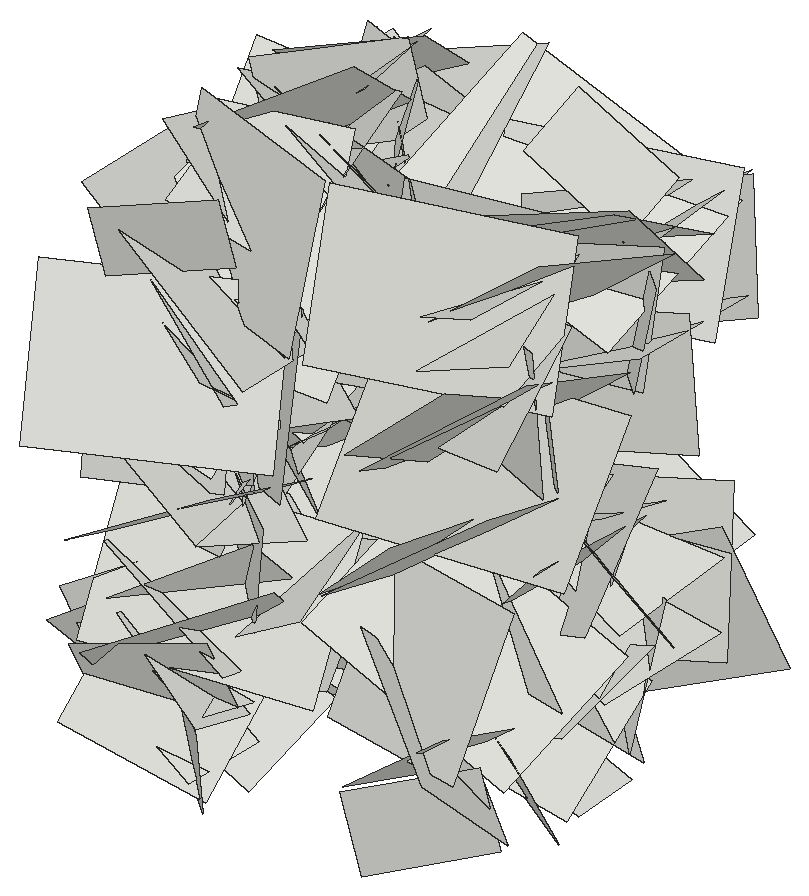
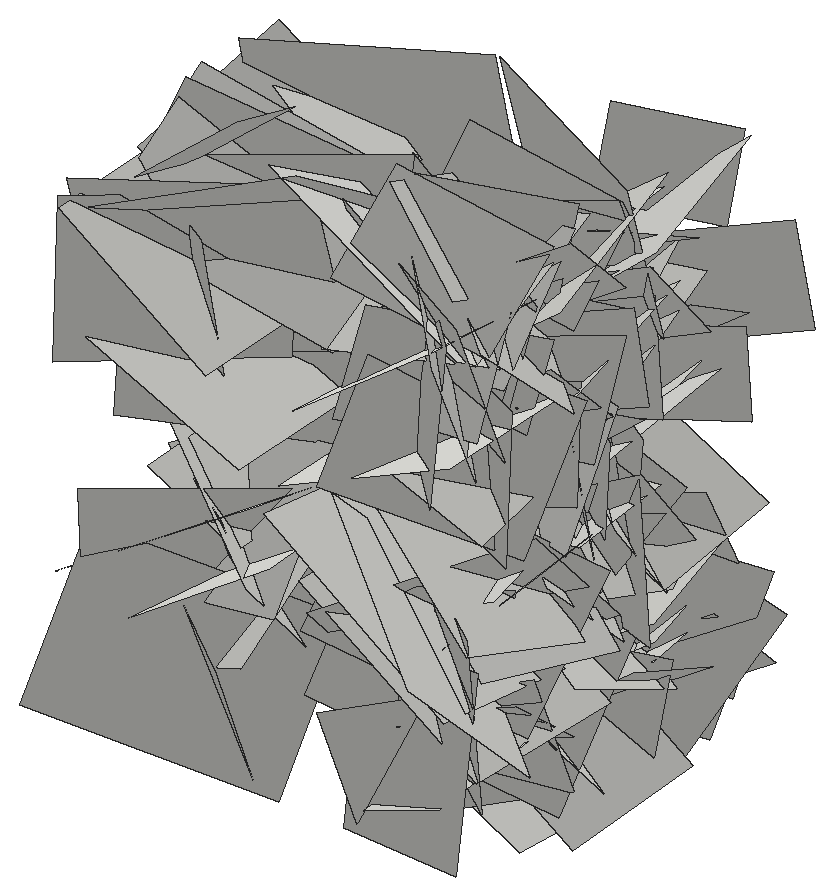
# SketchUp Ruby script. Lengths in inches.
U = 1.inch
M = Sketchup.active_model
def pt(a) = Geom::Point3d.new(a.map { |v| v * U })
def face(e, loops, mat)
  f = e.add_face(loops[0].map { |a| pt(a) })
  loops[1..].each { |l| e.add_face(l.map { |a| pt(a) }).erase! }
  f.material = f.back_material = mat if mat
  f
end
# faces: each face lists its corners as indices into pts; further lists are holes
def faces(e, pts, list, mat = nil) = list.each { |f| face(e, (f[0].is_a?(Array) ? f : [f]).map { |l| l.map { |i| pts[i] } }, mat) }
# xy, xz, yz: faces in a plane at the given z, y or x. An outline is a flat list of corners, or four numbers for a rectangle; further outlines are holes
def ring(l) = l.size == 4 ? [[l[0], l[1]], [l[2], l[1]], [l[2], l[3]], [l[0], l[3]]] : l.each_slice(2).to_a
def flat(e, list, mat, &to3) = list.each { |f| face(e, (f[0].is_a?(Array) ? f : [f]).map { |l| ring(l).map { |u, v| to3.(u, v) } }, mat) }
def xy(e, z, list, mat = nil) = flat(e, list, mat) { |x, y| [x, y, z] }
def xz(e, y, list, mat = nil) = flat(e, list, mat) { |x, z| [x, y, z] }
def yz(e, x, list, mat = nil) = flat(e, list, mat) { |y, z| [x, y, z] }
def lines(e, pts, list) = list.each { |a, b| e.add_line(pt(pts[a]), pt(pts[b])) }
# prism: a flat outline (further loops are holes) pulled along v
def prism(e, loops, v, mat = nil)
  f = face(e, loops, mat); d = Geom::Vector3d.new(v.map { |x| x * U })
  f.pushpull(f.normal.samedirection?(d) ? d.length : -d.length)
end
def box(e, o, s, mat = nil) = prism(e, [[o, [o[0] + s[0], o[1], o[2]], [o[0] + s[0], o[1] + s[1], o[2]], [o[0], o[1] + s[1], o[2]]]], [0, 0, s[2]], mat)
def at(x, y, z, deg = 0) = Geom::Transformation.translation(pt([x, y, z])) * Geom::Transformation.rotation(ORIGIN, Z_AXIS, deg.degrees)
def axes(o, x, y, z) = Geom::Transformation.new([*x, 0, *y, 0, *z, 0, *pt(o).to_a, 1])
def part(name) = M.definitions.add(name)
# library, detail: a bought-in or finely detailed component or shape, given as its bounding box
def library(name, o, s) = part(name).tap { |d| box(d.entities, o, s) }
def detail(e, o, s) = box(e.add_group.entities, o, s)
def put(e, d, t, mat = nil) = e.add_instance(d, t).tap { |i| i.material = mat if mat }
def group(e, t, mat = nil) = e.add_group.tap { |g| g.transformation = t; g.material = mat if mat }.entities
root = M.entities
c1 = part("Component\#6")
p = [[0.01,0,0],[0,3.24,4.54],[4.32,3.24,4.54],[4.33,0,0]]
faces(c1.entities,p,[[0,1,2,3]])
put(root,c1,axes([24.34,175.72,36.8],[-0.15665,0.75943,0.7145],[-0.11122,0.70715,-0.77331],[1.09966,0.17971,0.02357]))
put(root,c1,axes([28.31,175.72,36.8],[0.15665,0.75943,0.7145],[0.11122,0.70715,-0.77331],[-1.09966,0.17971,0.02357]))
put(root,c1,axes([24.34,182.09,31.375],[0.0562,-0.72005,0.10613],[0.07977,0.11126,0.71729],[0.76737,0.04117,-0.08234]))
put(root,c1,axes([28.31,170.91,25.11],[-0.00896,0.33986,-0.6335],[-0.15678,-0.62081,-0.33108],[-0.74574,0.12644,0.07722]))
put(root,c1,axes([28.31,181.67,36.78],[0.05967,0.56874,-0.94691],[0.29528,-0.9248,-0.5389],[-1.13301,-0.21107,-0.19031]))
put(root,c1,axes([28.31,180.66,33.34],[0.08177,-0.45253,0.73357],[-0.03972,0.73405,0.45677],[-0.91278,-0.07248,0.04584]))
put(root,c1,axes([24.34,176.52,27.27],[0.06139,-0.83333,-0.30669],[-0.14477,-0.31205,0.82208],[0.93005,0.00643,0.1482]))
put(root,c1,axes([24.34,174.67,32.54],[-0.17055,0.3665,0.95024],[-0.03456,0.95968,-0.37566],[1.07902,0.08867,0.13816]))
put(root,c1,axes([24.34,177.99,23.55],[0.04107,0.5427,0.4395],[0.20397,0.41484,-0.52921],[0.71159,-0.15024,0.12632]))
put(root,c1,axes([24.34,177.89,30.77],[0.05678,-0.11721,0.8526],[-0.09083,0.84928,0.12214],[0.90772,0.09231,-0.04111]))
put(root,c1,axes([24.34,174.875,32.24],[0.12053,0.70886,0.38052],[-0.08644,0.39248,-0.70676],[0.84842,-0.06072,-0.12606]))
put(root,c1,axes([24.34,176.26,32.94],[0.03084,0.60524,0.59943],[-0.03406,0.60013,-0.60439],[0.90231,0.00196,-0.0433]))
put(root,c1,axes([24.34,169.05,21.98],[0.04882,0.58162,0.59704],[-0.02934,0.59868,-0.58109],[0.88303,-0.01226,-0.05232]))
put(root,c1,axes([24.34,171.18,26.98],[-0.09963,0.88743,-0.23237],[0.05305,-0.22828,-0.89204],[0.97094,0.10354,0.02489]))
put(root,c1,axes([24.34,174.16,29.86],[0.19319,0.59277,-0.26834],[0.07097,-0.29428,-0.60458],[0.68606,-0.13648,0.1381]))
put(root,c1,axes([28.31,171.52,27.71],[0.03995,0.48298,0.66079],[0.01207,0.66111,-0.48387],[-0.8675,0.03144,0.0237]))
put(root,c1,axes([24.34,174.95,31.63],[0.12097,-0.07785,-0.70642],[0.09105,-0.70871,0.09198],[0.74781,0.09888,0.10307]))
put(root,c1,axes([24.34,178.01,36.42],[0.04909,-0.68925,0.58112],[-0.09024,0.57594,0.68989],[0.95135,0.0902,0.03545]))
put(root,c1,axes([24.34,172,20.82],[-0.19013,-0.4174,1.11707],[-0.18593,1.12659,0.39279],[1.25031,0.10406,0.22828]))
put(root,c1,axes([28.31,172.01,32.68],[-0.01531,-0.04852,-0.71126],[-0.05574,-0.70939,0.04946],[-0.75363,0.05345,0.01079]))
put(root,c1,axes([24.34,184.3,37.98],[-0.01849,-0.42221,-1.00939],[-0.24573,-0.98518,0.41609],[1.13346,-0.22047,0.07374]))
put(root,c1,axes([24.34,175.14,30.45],[-0.22771,0.17317,-1.07869],[0.0194,-1.09862,-0.18001],[1.15789,0.05246,-0.20912]))
put(root,c1,axes([28.31,173.36,27.66],[0.12062,0.63946,0.63128],[0.06443,0.62939,-0.6485],[-0.9503,0.12384,0.03616]))
put(root,c1,axes([28.31,173.29,20.87],[-0.09428,-0.62013,-0.08152],[-0.03551,-0.0775,0.6261],[-0.66205,0.09247,-0.02197]))
put(root,c1,axes([24.34,180.04,24.28],[0.15161,0.71603,-0.23582],[0.04269,-0.24694,-0.72538],[0.79796,-0.12284,0.08362]))
put(root,c1,axes([24.34,178.05,19.9375],[-0.14578,-1.0409,0.22357],[-0.02192,0.228,1.04879],[1.1283,-0.13006,0.04926]))
put(root,c1,axes([24.34,171.36,22.89],[0.02535,0.88672,0.32576],[-0.06435,0.32663,-0.88464],[0.99927,-0.00146,-0.06523]))
put(root,c1,axes([24.34,176.41,32.2],[0.11408,-0.0942,-0.79779],[0.0272,-0.8041,0.09841],[0.85109,0.03832,0.10379]))
put(root,c1,axes([28.31,177.7,39.03],[0.08239,-0.33737,-0.64844],[-0.10668,-0.65083,0.32654],[-0.76743,0.05425,-0.11501]))
put(root,c1,axes([24.34,181.8125,37.17],[-0.0246,-0.63961,0.56311],[0.17949,0.54862,0.63013],[0.88529,-0.129,-0.11211]))
put(root,c1,axes([24.34,173.5,20.5],[-0.29119,-0.77592,0.90535],[0.00734,0.92801,0.79744],[1.26387,-0.18415,0.20396]))
put(root,c1,axes([24.34,172.625,27.43],[-0.01975,0.58315,0.74345],[0.01761,0.74368,-0.58292],[1.00141,-0.00157,0.02491]))
put(root,c1,axes([24.34,172.13,35.78],[0.07615,0.65901,-0.5201],[0.04859,-0.52431,-0.658],[0.88857,-0.02781,0.08055]))
put(root,c1,axes([24.34,177.13,31.79],[-0.078,-0.30439,1.03044],[-0.07955,1.03178,0.29943],[1.13614,0.05135,0.09171]))
put(root,c1,axes([24.34,182.1,27.04],[-0.18817,-1.1788,-0.21223],[-0.10509,-0.19936,1.19019],[1.26526,-0.19187,0.06729]))
put(root,c1,axes([28.31,180.11,41],[0.0874,0.13713,-0.78202],[0.02965,-0.78624,-0.13492],[-0.84107,-0.01347,-0.08602]))
put(root,c1,axes([28.31,171.42,39.46],[-0.01769,0.21401,-0.61924],[-0.03571,-0.6189,-0.21298],[-0.69357,0.02641,0.02676]))
put(root,c1,axes([28.31,174.375,32.02],[0.18574,0.64681,-0.5499],[0.00393,-0.56207,-0.65994],[-0.8999,0.13105,-0.11638]))
put(root,c1,axes([24.34,167.34,31.77],[-0.2501,0.51374,1.1242],[-0.05799,1.13903,-0.532],[1.3089,0.14863,0.19123]))
put(root,c1,axes([28.31,173.15,22.23],[-0.01199,-0.5915,0.12784],[-0.10227,0.12799,0.58366],[-0.63327,-0.00947,-0.09668]))
put(root,c1,axes([24.34,170.16,39.2],[-0.24703,1.2789,-0.21613],[-0.13589,-0.24123,-1.28918],[1.36812,0.20696,-0.16707]))
put(root,c1,axes([24.34,174.01,26.46],[-0.07872,-0.97306,0.24072],[0.0738,0.23579,0.97461],[1.05998,-0.08868,-0.04998]))
put(root,c1,axes([28.31,173.67,32.24],[0.05341,-0.65994,-0.37026],[0.06447,-0.36634,0.66124],[-0.79951,-0.07362,0.02859]))
put(root,c1,axes([28.31,175.43,34.87],[0.0411,0.62613,0.35799],[0.03637,0.3565,-0.62724],[-0.76365,0.05068,-0.01061]))
put(root,c1,axes([24.34,185.38,28.27],[-0.28552,-0.8956,-0.93898],[-0.07116,-0.9481,0.92355],[1.37362,-0.23528,-0.14733]))
put(root,c1,axes([24.34,182.77,28.15],[-0.11013,-1.0722,-0.31704],[-0.03816,-0.31503,1.07721],[1.18456,-0.10983,0.00522]))
put(root,c1,axes([24.34,176.05,33.17],[0.01986,0.50916,-0.88553],[-0.06176,-0.8837,-0.50934],[1.08099,-0.05984,-0.01283]))
put(root,c1,axes([28.31,182.27,37.76],[0.22679,0.05489,-0.89691],[0.06736,-0.9206,-0.04118],[-0.95012,-0.05216,-0.217]))
put(root,c1,axes([24.34,174.9,23.69],[-0.06803,0.90477,0.33383],[0.16872,0.33992,-0.89067],[1.00823,0.00417,0.17157]))
put(root,c1,axes([28.31,173.11,21.9],[0.05319,-0.68826,0.19248],[0.04456,0.19546,0.68797],[-0.75624,-0.03689,0.05408]))
put(root,c1,axes([28.31,178.15,33.23],[-0.08938,-0.00525,-0.60269],[0.06829,-0.60515,-0.00374],[-0.63521,-0.06432,0.0844]))
put(root,c1,axes([28.31,176.44,21.6],[0.04345,0.60879,-0.00304],[-0.10651,0.00376,-0.60183],[-0.63647,0.04093,0.10051]))
put(root,c1,axes([24.34,183.67,38.38],[0.04708,0.10578,-1.15378],[-0.2342,-1.13267,-0.11235],[1.2056,-0.22416,0.02323]))
put(root,c1,axes([24.34,173.31,35.98],[-0.01252,1.07454,-0.37217],[-0.12805,-0.37127,-1.06811],[1.19858,-0.02844,-0.11799]))
put(root,c1,axes([24.34,174.78,20.26],[0.10048,-0.39109,0.79293],[0.10042,0.79738,0.38196],[0.93179,-0.04376,-0.12667]))
put(root,c1,axes([28.31,180.68,27.18],[0.06604,-0.60003,0.10008],[-0.10227,0.08959,0.59716],[-0.63666,-0.07663,-0.08554]))
put(root,c1,axes([28.31,170.73,19.61],[0.06378,-0.15247,0.68566],[0.07422,0.68605,0.14641],[-0.74085,0.05561,0.0737]))
put(root,c1,axes([24.34,178.01,21.81],[0.00864,0.40014,0.99077],[-0.02339,0.99065,-0.39991],[1.13239,0.01741,-0.01582]))
put(root,c1,axes([28.31,178.13,40.15],[0.04908,0.64392,0.19174],[0.08573,0.18545,-0.64234],[-0.70699,0.06719,-0.06458]))
put(root,c1,axes([24.34,171.95,33.74],[-0.07102,0.70639,0.8167],[0.11892,0.8184,-0.69866],[1.13841,-0.04142,0.12393]))
put(root,c1,axes([28.31,176.07,37.03],[0.15674,-0.62528,-0.09698],[-0.10666,-0.12156,0.63036],[-0.66219,-0.12843,-0.12449]))
put(root,c1,axes([28.31,180.42,25.12],[0.17902,-0.88337,-0.09354],[0.21931,-0.05348,0.8786],[-0.91571,-0.1855,0.19214]))
put(root,c1,axes([24.34,172.46,21.25],[0.14489,-0.73421,0.72244],[-0.08794,0.71856,0.74596],[1.0883,0.15581,-0.0359]))
put(root,c1,axes([24.34,171.47,32.36],[0.16942,0.96147,-0.31887],[-0.08969,-0.30901,-0.97416],[1.06999,-0.17814,-0.03117]))
put(root,c1,axes([24.34,179.35,38.14],[0.07028,1.07405,0.02302],[-0.04111,0.02544,-1.07534],[1.13802,-0.06541,-0.04027]))
put(root,c1,axes([28.31,181.39,28.46],[0.11732,-0.15238,-0.58962],[-0.01785,-0.59981,0.15186],[-0.64528,-0.01111,-0.1114]))
put(root,c1,axes([28.31,173.74,31.89],[0.15856,-0.67469,0.29232],[0.1064,0.31425,0.67394],[-0.77211,-0.09525,0.1529]))
put(root,c1,axes([24.34,173.84,39.64],[-0.13369,1.27699,-0.41872],[-0.11509,-0.42887,-1.27523],[1.41986,0.08547,-0.14279]))
put(root,c1,axes([28.31,172.58,29],[0.14706,-0.68518,0.03236],[0.10474,0.05263,0.69082],[-0.71951,-0.13238,0.10718]))
put(root,c1,axes([24.34,180.75,35.09],[-0.01445,0.08276,-1.11066],[0.1396,-1.10283,-0.0838],[1.17228,0.13235,-0.00371]))
put(root,c1,axes([24.34,182.25,27.43],[-0.1955,0.46825,-1.21407],[0.10064,-1.21809,-0.48422],[1.37564,0.15566,-0.13711]))
put(root,c1,axes([24.34,175.96,26.52],[0.03553,0.82214,0.9074],[-0.07429,0.90754,-0.81968],[1.2958,0.02948,-0.07187]))
put(root,c1,axes([24.34,172.47,36.95],[0.1233,0.89549,0.4145],[0.21728,0.38634,-0.89217],[1.02316,-0.18996,0.13951]))
put(root,c1,axes([24.34,183.25,38.77],[-0.07927,-0.40868,-1.12281],[0.1988,-1.11508,0.39337],[1.25087,0.15132,-0.13368]))
put(root,c1,axes([24.34,179.04,23.77],[0.11323,-0.75693,-0.7774],[0.09292,-0.77258,0.76428],[1.14637,0.13739,0.01483]))
put(root,c1,axes([24.34,182.77,28.7],[-0.0358,-0.11408,-1.31406],[-0.04325,-1.31377,0.1151],[1.39747,-0.04358,-0.0301]))
put(root,c1,axes([24.34,180.07,24.39],[-0.06666,-0.76105,0.92501],[0.21989,0.90537,0.75899],[1.25053,-0.19976,-0.08415]))
put(root,c1,axes([24.34,177.97,39.67],[-0.02985,0.75948,-0.84861],[0.27983,-0.8214,-0.74388],[1.17429,0.21504,0.15569]))
put(root,c1,axes([24.34,174.06,31.875],[0.08593,-0.00736,1.08266],[0.18405,1.07173,-0.00571],[1.1328,-0.17357,-0.0812]))
put(root,c1,axes([24.34,182.31,23.94],[-0.04872,-1.30982,0.04089],[0.01644,0.04037,1.31055],[1.38898,-0.04642,-0.01408]))
put(root,c1,axes([24.34,178.49,34.59],[0.00763,1.14917,-0.03145],[0.21412,-0.03223,-1.13128],[1.19962,-0.00155,0.20212]))
put(root,c1,axes([24.34,178.09,32.9],[0.18757,-0.47698,-1.21124],[-0.23196,-1.21588,0.44684],[1.36024,-0.14157,0.24323]))
put(root,c1,axes([24.34,178.68,21.25],[0.14964,-1.02559,0.91665],[-0.24358,0.89093,1.03221],[1.43757,0.25771,0.07948]))
put(root,c1,axes([24.34,169.91,24.28],[-0.0494,0.58776,1.07494],[0.25393,1.05932,-0.56884],[1.27358,-0.18841,0.15511]))
put(root,c1,axes([24.34,175.66,39.88],[-0.03914,-0.32872,-1.22009],[0.25418,-1.20026,0.31612],[1.31508,0.2222,-0.09741]))
put(root,c1,axes([24.34,177.96,25.04],[0.10915,-1.1796,-0.55067],[0.03689,-0.5497,1.18402],[1.37942,0.10803,0.01191]))
put(root,c1,axes([24.34,183.77,26.5],[0.0762,-1.33255,-0.21023],[0.04546,-0.20817,1.33413],[1.42926,0.07766,-0.03122]))
put(root,c1,axes([24.34,177.28,39.83],[0.04784,1.11638,-0.64936],[0.22797,-0.64718,-1.09769],[1.34988,0.06974,0.20839]))
put(root,c1,axes([24.34,179.625,37.91],[0.28026,0.12179,-1.29213],[0.26115,-1.29941,-0.07206],[1.35072,0.22596,0.28204]))
put(root,c1,axes([24.34,183.19,37.72],[0.19709,-1.17807,-0.70591],[0.26547,-0.67132,1.18631],[1.43137,0.28672,-0.12282]))
put(root,c1,axes([38.11,183.19,37.72],[-0.19709,-1.17807,-0.70591],[-0.26547,-0.67132,1.18631],[-1.43137,0.28672,-0.12282]))
put(root,c1,axes([38.11,179.625,37.91],[-0.28026,0.12179,-1.29213],[-0.26115,-1.29941,-0.07206],[-1.35072,0.22596,0.28204]))
put(root,c1,axes([38.11,177.28,39.83],[-0.04784,1.11638,-0.64936],[-0.22797,-0.64718,-1.09769],[-1.34988,0.06974,0.20839]))
put(root,c1,axes([38.11,183.77,26.5],[-0.0762,-1.33255,-0.21023],[-0.04546,-0.20817,1.33413],[-1.42926,0.07766,-0.03122]))
put(root,c1,axes([38.11,177.96,25.04],[-0.10915,-1.1796,-0.55067],[-0.03689,-0.5497,1.18402],[-1.37942,0.10803,0.01191]))
put(root,c1,axes([38.11,175.66,39.88],[0.03914,-0.32872,-1.22009],[-0.25418,-1.20026,0.31612],[-1.31508,0.2222,-0.09741]))
put(root,c1,axes([38.11,169.91,24.28],[0.0494,0.58776,1.07494],[-0.25393,1.05932,-0.56884],[-1.27358,-0.18841,0.15511]))
put(root,c1,axes([38.11,178.68,21.25],[-0.14964,-1.02559,0.91665],[0.24358,0.89093,1.03221],[-1.43757,0.25771,0.07948]))
put(root,c1,axes([38.11,178.09,32.9],[-0.18757,-0.47698,-1.21124],[0.23196,-1.21588,0.44684],[-1.36024,-0.14157,0.24323]))
put(root,c1,axes([38.11,178.49,34.59],[-0.00763,1.14917,-0.03145],[-0.21412,-0.03223,-1.13128],[-1.19962,-0.00155,0.20212]))
put(root,c1,axes([38.11,182.31,23.94],[0.04872,-1.30982,0.04089],[-0.01644,0.04037,1.31055],[-1.38898,-0.04642,-0.01408]))
put(root,c1,axes([38.11,174.06,31.875],[-0.08593,-0.00736,1.08266],[-0.18405,1.07173,-0.00571],[-1.1328,-0.17357,-0.0812]))
put(root,c1,axes([38.11,177.97,39.67],[0.02985,0.75948,-0.84861],[-0.27983,-0.8214,-0.74388],[-1.17429,0.21504,0.15569]))
put(root,c1,axes([38.11,180.07,24.39],[0.06666,-0.76105,0.92501],[-0.21989,0.90537,0.75899],[-1.25053,-0.19976,-0.08415]))
put(root,c1,axes([38.11,182.77,28.7],[0.0358,-0.11408,-1.31406],[0.04325,-1.31377,0.1151],[-1.39747,-0.04358,-0.0301]))
put(root,c1,axes([38.11,179.04,23.77],[-0.11323,-0.75693,-0.7774],[-0.09292,-0.77258,0.76428],[-1.14637,0.13739,0.01483]))
put(root,c1,axes([38.11,183.25,38.77],[0.07927,-0.40868,-1.12281],[-0.1988,-1.11508,0.39337],[-1.25087,0.15132,-0.13368]))
put(root,c1,axes([38.11,172.47,36.95],[-0.1233,0.89549,0.4145],[-0.21728,0.38634,-0.89217],[-1.02316,-0.18996,0.13951]))
put(root,c1,axes([38.11,175.96,26.52],[-0.03553,0.82214,0.9074],[0.07429,0.90754,-0.81968],[-1.2958,0.02948,-0.07187]))
put(root,c1,axes([38.11,182.25,27.43],[0.1955,0.46825,-1.21407],[-0.10064,-1.21809,-0.48422],[-1.37564,0.15566,-0.13711]))
put(root,c1,axes([38.11,180.75,35.09],[0.01445,0.08276,-1.11066],[-0.1396,-1.10283,-0.0838],[-1.17228,0.13235,-0.00371]))
put(root,c1,axes([34.14,172.58,29],[-0.14706,-0.68518,0.03236],[-0.10474,0.05263,0.69082],[0.71951,-0.13238,0.10718]))
put(root,c1,axes([38.11,173.84,39.64],[0.13369,1.27699,-0.41872],[0.11509,-0.42887,-1.27523],[-1.41986,0.08547,-0.14279]))
put(root,c1,axes([34.14,173.74,31.89],[-0.15856,-0.67469,0.29232],[-0.1064,0.31425,0.67394],[0.77211,-0.09525,0.1529]))
put(root,c1,axes([34.14,181.39,28.46],[-0.11732,-0.15238,-0.58962],[0.01785,-0.59981,0.15186],[0.64528,-0.01111,-0.1114]))
put(root,c1,axes([38.11,179.35,38.14],[-0.07028,1.07405,0.02302],[0.04111,0.02544,-1.07534],[-1.13802,-0.06541,-0.04027]))
put(root,c1,axes([38.11,171.47,32.36],[-0.16942,0.96147,-0.31887],[0.08969,-0.30901,-0.97416],[-1.06999,-0.17814,-0.03117]))
put(root,c1,axes([38.11,172.46,21.25],[-0.14489,-0.73421,0.72244],[0.08794,0.71856,0.74596],[-1.0883,0.15581,-0.0359]))
put(root,c1,axes([34.14,180.42,25.12],[-0.17902,-0.88337,-0.09354],[-0.21931,-0.05348,0.8786],[0.91571,-0.1855,0.19214]))
put(root,c1,axes([34.14,176.07,37.03],[-0.15674,-0.62528,-0.09698],[0.10666,-0.12156,0.63036],[0.66219,-0.12843,-0.12449]))
put(root,c1,axes([38.11,171.95,33.74],[0.07102,0.70639,0.8167],[-0.11892,0.8184,-0.69866],[-1.13841,-0.04142,0.12393]))
put(root,c1,axes([34.14,178.13,40.15],[-0.04908,0.64392,0.19174],[-0.08573,0.18545,-0.64234],[0.70699,0.06719,-0.06458]))
put(root,c1,axes([38.11,178.01,21.81],[-0.00864,0.40014,0.99077],[0.02339,0.99065,-0.39991],[-1.13239,0.01741,-0.01582]))
put(root,c1,axes([34.14,170.73,19.61],[-0.06378,-0.15247,0.68566],[-0.07422,0.68605,0.14641],[0.74085,0.05561,0.0737]))
put(root,c1,axes([34.14,180.68,27.18],[-0.06604,-0.60003,0.10008],[0.10227,0.08959,0.59716],[0.63666,-0.07663,-0.08554]))
put(root,c1,axes([38.11,174.78,20.26],[-0.10048,-0.39109,0.79293],[-0.10042,0.79738,0.38196],[-0.93179,-0.04376,-0.12667]))
put(root,c1,axes([38.11,173.31,35.98],[0.01252,1.07454,-0.37217],[0.12805,-0.37127,-1.06811],[-1.19858,-0.02844,-0.11799]))
put(root,c1,axes([38.11,183.67,38.38],[-0.04708,0.10578,-1.15378],[0.2342,-1.13267,-0.11235],[-1.2056,-0.22416,0.02323]))
put(root,c1,axes([34.14,176.44,21.6],[-0.04345,0.60879,-0.00304],[0.10651,0.00376,-0.60183],[0.63647,0.04093,0.10051]))
put(root,c1,axes([34.14,178.15,33.23],[0.08938,-0.00525,-0.60269],[-0.06829,-0.60515,-0.00374],[0.63521,-0.06432,0.0844]))
put(root,c1,axes([34.14,173.11,21.9],[-0.05319,-0.68826,0.19248],[-0.04456,0.19546,0.68797],[0.75624,-0.03689,0.05408]))
put(root,c1,axes([38.11,174.9,23.69],[0.06803,0.90477,0.33383],[-0.16872,0.33992,-0.89067],[-1.00823,0.00417,0.17157]))
put(root,c1,axes([34.14,182.27,37.76],[-0.22679,0.05489,-0.89691],[-0.06736,-0.9206,-0.04118],[0.95012,-0.05216,-0.217]))
